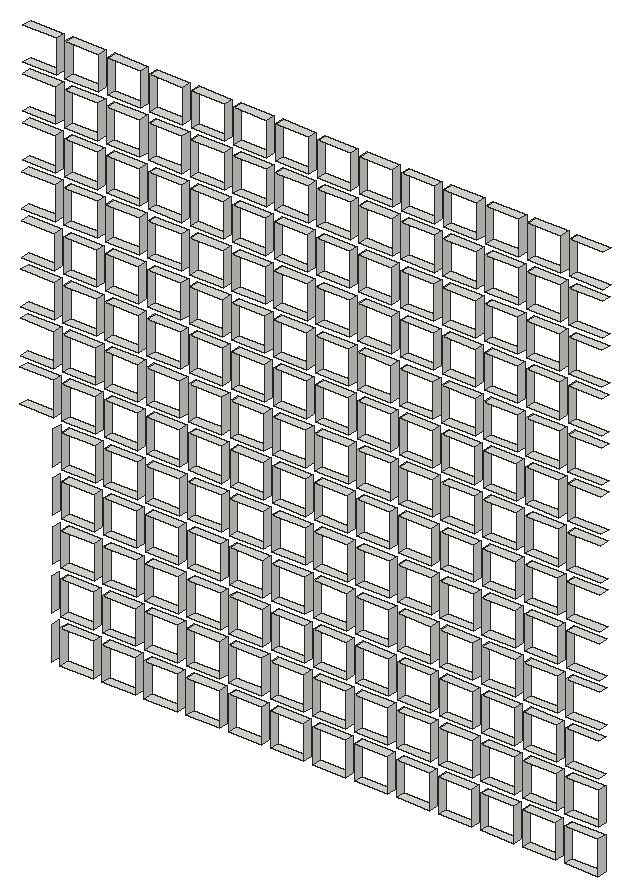
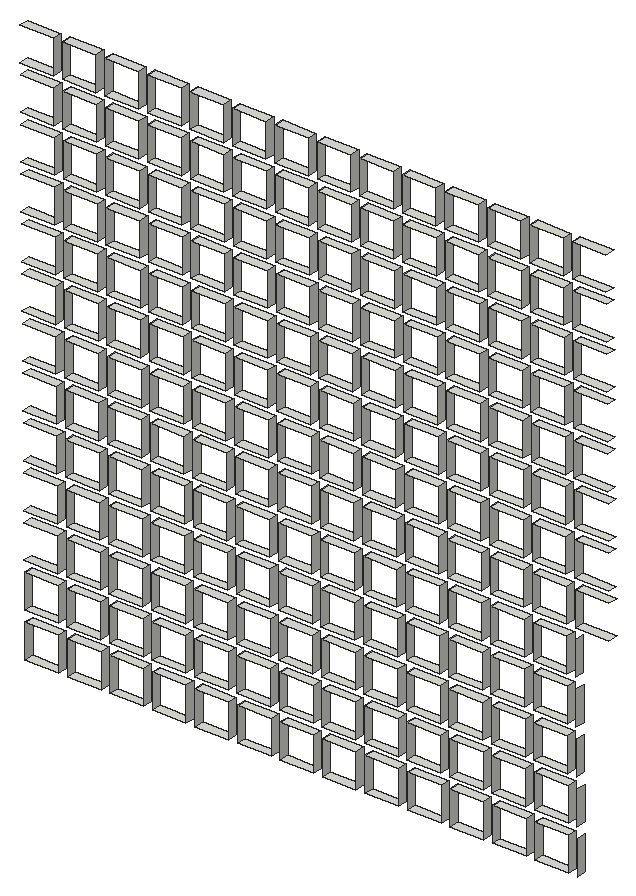
# SketchUp Ruby script. Lengths in inches.
U = 1.inch
M = Sketchup.active_model
def pt(a) = Geom::Point3d.new(a.map { |v| v * U })
def face(e, loops, mat)
  f = e.add_face(loops[0].map { |a| pt(a) })
  loops[1..].each { |l| e.add_face(l.map { |a| pt(a) }).erase! }
  f.material = f.back_material = mat if mat
  f
end
# faces: each face lists its corners as indices into pts; further lists are holes
def faces(e, pts, list, mat = nil) = list.each { |f| face(e, (f[0].is_a?(Array) ? f : [f]).map { |l| l.map { |i| pts[i] } }, mat) }
# xy, xz, yz: faces in a plane at the given z, y or x. An outline is a flat list of corners, or four numbers for a rectangle; further outlines are holes
def ring(l) = l.size == 4 ? [[l[0], l[1]], [l[2], l[1]], [l[2], l[3]], [l[0], l[3]]] : l.each_slice(2).to_a
def flat(e, list, mat, &to3) = list.each { |f| face(e, (f[0].is_a?(Array) ? f : [f]).map { |l| ring(l).map { |u, v| to3.(u, v) } }, mat) }
def xy(e, z, list, mat = nil) = flat(e, list, mat) { |x, y| [x, y, z] }
def xz(e, y, list, mat = nil) = flat(e, list, mat) { |x, z| [x, y, z] }
def yz(e, x, list, mat = nil) = flat(e, list, mat) { |y, z| [x, y, z] }
def lines(e, pts, list) = list.each { |a, b| e.add_line(pt(pts[a]), pt(pts[b])) }
# prism: a flat outline (further loops are holes) pulled along v
def prism(e, loops, v, mat = nil)
  f = face(e, loops, mat); d = Geom::Vector3d.new(v.map { |x| x * U })
  f.pushpull(f.normal.samedirection?(d) ? d.length : -d.length)
end
def box(e, o, s, mat = nil) = prism(e, [[o, [o[0] + s[0], o[1], o[2]], [o[0] + s[0], o[1] + s[1], o[2]], [o[0], o[1] + s[1], o[2]]]], [0, 0, s[2]], mat)
def at(x, y, z, deg = 0) = Geom::Transformation.translation(pt([x, y, z])) * Geom::Transformation.rotation(ORIGIN, Z_AXIS, deg.degrees)
def axes(o, x, y, z) = Geom::Transformation.new([*x, 0, *y, 0, *z, 0, *pt(o).to_a, 1])
def part(name) = M.definitions.add(name)
# library, detail: a bought-in or finely detailed component or shape, given as its bounding box
def library(name, o, s) = part(name).tap { |d| box(d.entities, o, s) }
def detail(e, o, s) = box(e.add_group.entities, o, s)
def put(e, d, t, mat = nil) = e.add_instance(d, t).tap { |i| i.material = mat if mat }
def group(e, t, mat = nil) = e.add_group.tap { |g| g.transformation = t; g.material = mat if mat }.entities
root = M.entities
xy(root,265.77,[[2217.37,480.14,2219.68,480.77],[2220.28,480.14,2222.59,480.77],[2223.19,480.14,2225.5,480.77],[2226.1,480.14,2228.42,480.77],[2229.02,480.14,2231.33,480.77],
  [2231.93,480.14,2234.24,480.77],[2234.84,480.14,2237.15,480.77],[2237.75,480.14,2240.06,480.77],[2240.66,480.14,2242.98,480.77],[2243.58,480.14,2245.89,480.77],
  [2246.49,480.14,2248.8,480.77],[2249.4,480.14,2251.71,480.77],[2252.3125,480.14,2254.625,480.77]])
xy(root,268.09,[[2217.37,480.14,2219.68,480.77],[2220.28,480.14,2222.59,480.77],[2223.19,480.14,2225.5,480.77],[2226.1,480.14,2228.42,480.77],[2229.02,480.14,2231.33,480.77],
  [2231.93,480.14,2234.24,480.77],[2234.84,480.14,2237.15,480.77],[2237.75,480.14,2240.06,480.77],[2240.66,480.14,2242.98,480.77],[2243.58,480.14,2245.89,480.77],
  [2246.49,480.14,2248.8,480.77],[2249.4,480.14,2251.71,480.77],[2252.3125,480.14,2254.625,480.77]])
xy(root,268.82,[[2217.4,480.14,2219.71,480.77],[2220.31,480.14,2222.62,480.77],[2223.22,480.14,2225.53,480.77],[2226.13,480.14,2228.45,480.77],[2229.05,480.14,2231.36,480.77],
  [2231.96,480.14,2234.27,480.77],[2234.87,480.14,2237.18,480.77],[2237.78,480.14,2240.09,480.77],[2240.69,480.14,2243.01,480.77],[2243.61,480.14,2245.92,480.77],
  [2246.52,480.14,2248.83,480.77],[2249.43,480.14,2251.74,480.77],[2252.34,480.14,2254.65,480.77]])
xy(root,271.13,[[2217.4,480.14,2219.71,480.77],[2220.31,480.14,2222.62,480.77],[2223.22,480.14,2225.53,480.77],[2226.13,480.14,2228.45,480.77],[2229.05,480.14,2231.36,480.77],
  [2231.96,480.14,2234.27,480.77],[2234.87,480.14,2237.18,480.77],[2237.78,480.14,2240.09,480.77],[2240.69,480.14,2243.01,480.77],[2243.61,480.14,2245.92,480.77],
  [2246.52,480.14,2248.83,480.77],[2249.43,480.14,2251.74,480.77],[2252.34,480.14,2254.65,480.77]])
xy(root,271.86,[[2217.43,480.14,2219.74,480.77],[2220.34,480.14,2222.65,480.77],[2223.25,480.14,2225.5625,480.77],[2226.16,480.14,2228.47,480.77],[2229.07,480.14,2231.39,480.77],
  [2231.99,480.14,2234.3,480.77],[2234.9,480.14,2237.21,480.77],[2237.81,480.14,2240.12,480.77],[2240.72,480.14,2243.03,480.77],[2243.63,480.14,2245.95,480.77],
  [2246.55,480.14,2248.86,480.77],[2249.46,480.14,2251.77,480.77],[2252.37,480.14,2254.68,480.77]])
xy(root,274.17,[[2217.43,480.14,2219.74,480.77],[2220.34,480.14,2222.65,480.77],[2223.25,480.14,2225.5625,480.77],[2226.16,480.14,2228.47,480.77],[2229.07,480.14,2231.39,480.77],
  [2231.99,480.14,2234.3,480.77],[2234.9,480.14,2237.21,480.77],[2237.81,480.14,2240.12,480.77],[2240.72,480.14,2243.03,480.77],[2243.63,480.14,2245.95,480.77],
  [2246.55,480.14,2248.86,480.77],[2249.46,480.14,2251.77,480.77],[2252.37,480.14,2254.68,480.77]])
xy(root,274.91,[[2217.46,480.14,2219.77,480.77],[2220.37,480.14,2222.68,480.77],[2223.28,480.14,2225.59,480.77],[2226.19,480.14,2228.5,480.77],[2229.1,480.14,2231.42,480.77],
  [2232.02,480.14,2234.33,480.77],[2234.93,480.14,2237.24,480.77],[2237.84,480.14,2240.15,480.77],[2240.75,480.14,2243.0625,480.77],[2243.66,480.14,2245.98,480.77],
  [2246.58,480.14,2248.89,480.77],[2249.49,480.14,2251.8,480.77],[2252.4,480.14,2254.71,480.77]])
xy(root,277.22,[[2217.46,480.14,2219.77,480.77],[2220.37,480.14,2222.68,480.77],[2223.28,480.14,2225.59,480.77],[2226.19,480.14,2228.5,480.77],[2229.1,480.14,2231.42,480.77],
  [2232.02,480.14,2234.33,480.77],[2234.93,480.14,2237.24,480.77],[2237.84,480.14,2240.15,480.77],[2240.75,480.14,2243.0625,480.77],[2243.66,480.14,2245.98,480.77],
  [2246.58,480.14,2248.89,480.77],[2249.49,480.14,2251.8,480.77],[2252.4,480.14,2254.71,480.77]])
xy(root,277.95,[[2217.48,480.14,2219.8,480.77],[2220.4,480.14,2222.71,480.77],[2223.31,480.14,2225.62,480.77],[2226.22,480.14,2228.53,480.77],[2229.13,480.14,2231.44,480.77],
  [2232.04,480.14,2234.36,480.77],[2234.96,480.14,2237.27,480.77],[2237.87,480.14,2240.18,480.77],[2240.78,480.14,2243.09,480.77],[2243.69,480.14,2246,480.77],
  [2246.6,480.14,2248.92,480.77],[2249.52,480.14,2251.83,480.77],[2252.43,480.14,2254.74,480.77]])
xy(root,280.26,[[2217.48,480.14,2219.8,480.77],[2220.4,480.14,2222.71,480.77],[2223.31,480.14,2225.62,480.77],[2226.22,480.14,2228.53,480.77],[2229.13,480.14,2231.44,480.77],
  [2232.04,480.14,2234.36,480.77],[2234.96,480.14,2237.27,480.77],[2237.87,480.14,2240.18,480.77],[2240.78,480.14,2243.09,480.77],[2243.69,480.14,2246,480.77],
  [2246.6,480.14,2248.92,480.77],[2249.52,480.14,2251.83,480.77],[2252.43,480.14,2254.74,480.77]])
xy(root,281,[[2214.6,480.14,2216.91,480.77],[2217.51,480.14,2219.83,480.77],[2220.43,480.14,2222.74,480.77],[2223.34,480.14,2225.65,480.77],[2226.25,480.14,2228.5625,480.77],
  [2229.16,480.14,2231.47,480.77],[2232.07,480.14,2234.39,480.77],[2234.99,480.14,2237.3,480.77],[2237.9,480.14,2240.21,480.77],[2240.81,480.14,2243.12,480.77],
  [2243.72,480.14,2246.03,480.77],[2246.63,480.14,2248.95,480.77],[2249.55,480.14,2251.86,480.77],[2252.46,480.14,2254.77,480.77]])
xy(root,283.31,[[2214.6,480.14,2216.91,480.77],[2217.51,480.14,2219.83,480.77],[2220.43,480.14,2222.74,480.77],[2223.34,480.14,2225.65,480.77],[2226.25,480.14,2228.5625,480.77],
  [2229.16,480.14,2231.47,480.77],[2232.07,480.14,2234.39,480.77],[2234.99,480.14,2237.3,480.77],[2237.9,480.14,2240.21,480.77],[2240.81,480.14,2243.12,480.77],
  [2243.72,480.14,2246.03,480.77],[2246.63,480.14,2248.95,480.77],[2249.55,480.14,2251.86,480.77],[2252.46,480.14,2254.77,480.77]])
xy(root,284.04,[[2214.63,480.14,2216.94,480.77],[2217.54,480.14,2219.85,480.77],[2220.45,480.14,2222.77,480.77],[2223.37,480.14,2225.68,480.77],[2226.28,480.14,2228.59,480.77],
  [2229.19,480.14,2231.5,480.77],[2232.1,480.14,2234.41,480.77],[2235.01,480.14,2237.33,480.77],[2237.93,480.14,2240.24,480.77],[2240.84,480.14,2243.15,480.77],
  [2243.75,480.14,2246.0625,480.77],[2246.66,480.14,2248.97,480.77],[2249.57,480.14,2251.89,480.77],[2252.49,480.14,2254.8,480.77]])
xy(root,286.35,[[2214.63,480.14,2216.94,480.77],[2217.54,480.14,2219.85,480.77],[2220.45,480.14,2222.77,480.77],[2223.37,480.14,2225.68,480.77],[2226.28,480.14,2228.59,480.77],
  [2229.19,480.14,2231.5,480.77],[2232.1,480.14,2234.41,480.77],[2235.01,480.14,2237.33,480.77],[2237.93,480.14,2240.24,480.77],[2240.84,480.14,2243.15,480.77],
  [2243.75,480.14,2246.0625,480.77],[2246.66,480.14,2248.97,480.77],[2249.57,480.14,2251.89,480.77],[2252.49,480.14,2254.8,480.77]])
xy(root,287.09,[[2214.66,480.14,2216.97,480.77],[2217.57,480.14,2219.88,480.77],[2220.48,480.14,2222.8,480.77],[2223.4,480.14,2225.71,480.77],[2226.31,480.14,2228.62,480.77],
  [2229.22,480.14,2231.53,480.77],[2232.13,480.14,2234.44,480.77],[2235.04,480.14,2237.36,480.77],[2237.96,480.14,2240.27,480.77],[2240.87,480.14,2243.18,480.77],
  [2243.78,480.14,2246.09,480.77],[2246.69,480.14,2249,480.77],[2249.6,480.14,2251.92,480.77],[2252.52,480.14,2254.83,480.77]])
xy(root,289.4,[[2214.66,480.14,2216.97,480.77],[2217.57,480.14,2219.88,480.77],[2220.48,480.14,2222.8,480.77],[2223.4,480.14,2225.71,480.77],[2226.31,480.14,2228.62,480.77],
  [2229.22,480.14,2231.53,480.77],[2232.13,480.14,2234.44,480.77],[2235.04,480.14,2237.36,480.77],[2237.96,480.14,2240.27,480.77],[2240.87,480.14,2243.18,480.77],
  [2243.78,480.14,2246.09,480.77],[2246.69,480.14,2249,480.77],[2249.6,480.14,2251.92,480.77],[2252.52,480.14,2254.83,480.77]])
xy(root,290.13,[[2214.6875,480.14,2217,480.77],[2217.6,480.14,2219.91,480.77],[2220.51,480.14,2222.82,480.77],[2223.42,480.14,2225.74,480.77],[2226.34,480.14,2228.65,480.77],
  [2229.25,480.14,2231.5625,480.77],[2232.16,480.14,2234.47,480.77],[2235.07,480.14,2237.38,480.77],[2237.98,480.14,2240.3,480.77],[2240.9,480.14,2243.21,480.77],
  [2243.81,480.14,2246.12,480.77],[2246.72,480.14,2249.03,480.77],[2249.63,480.14,2251.94,480.77],[2252.54,480.14,2254.86,480.77]])
xy(root,292.44,[[2214.6875,480.14,2217,480.77],[2217.6,480.14,2219.91,480.77],[2220.51,480.14,2222.82,480.77],[2223.42,480.14,2225.74,480.77],[2226.34,480.14,2228.65,480.77],
  [2229.25,480.14,2231.5625,480.77],[2232.16,480.14,2234.47,480.77],[2235.07,480.14,2237.38,480.77],[2237.98,480.14,2240.3,480.77],[2240.9,480.14,2243.21,480.77],
  [2243.81,480.14,2246.12,480.77],[2246.72,480.14,2249.03,480.77],[2249.63,480.14,2251.94,480.77],[2252.54,480.14,2254.86,480.77]])
xy(root,293.18,[[2214.72,480.14,2217.03,480.77],[2217.63,480.14,2219.94,480.77],[2220.54,480.14,2222.85,480.77],[2223.45,480.14,2225.77,480.77],[2226.37,480.14,2228.68,480.77],
  [2229.28,480.14,2231.59,480.77],[2232.1875,480.14,2234.5,480.77],[2235.1,480.14,2237.41,480.77],[2238.01,480.14,2240.33,480.77],[2240.93,480.14,2243.24,480.77],
  [2243.84,480.14,2246.15,480.77],[2246.75,480.14,2249.0625,480.77],[2249.66,480.14,2251.97,480.77],[2252.57,480.14,2254.89,480.77]])
xy(root,295.49,[[2214.72,480.14,2217.03,480.77],[2217.63,480.14,2219.94,480.77],[2220.54,480.14,2222.85,480.77],[2223.45,480.14,2225.77,480.77],[2226.37,480.14,2228.68,480.77],
  [2229.28,480.14,2231.59,480.77],[2232.1875,480.14,2234.5,480.77],[2235.1,480.14,2237.41,480.77],[2238.01,480.14,2240.33,480.77],[2240.93,480.14,2243.24,480.77],
  [2243.84,480.14,2246.15,480.77],[2246.75,480.14,2249.0625,480.77],[2249.66,480.14,2251.97,480.77],[2252.57,480.14,2254.89,480.77]])
xy(root,296.22,[[2214.75,480.14,2217.06,480.77],[2217.66,480.14,2219.97,480.77],[2220.57,480.14,2222.88,480.77],[2223.48,480.14,2225.79,480.77],[2226.39,480.14,2228.71,480.77],
  [2229.31,480.14,2231.62,480.77],[2232.22,480.14,2234.53,480.77],[2235.13,480.14,2237.44,480.77],[2238.04,480.14,2240.35,480.77],[2240.95,480.14,2243.27,480.77],
  [2243.87,480.14,2246.18,480.77],[2246.78,480.14,2249.09,480.77],[2249.69,480.14,2252,480.77],[2252.6,480.14,2254.91,480.77]])
xy(root,298.53,[[2214.75,480.14,2217.06,480.77],[2217.66,480.14,2219.97,480.77],[2220.57,480.14,2222.88,480.77],[2223.48,480.14,2225.79,480.77],[2226.39,480.14,2228.71,480.77],
  [2229.31,480.14,2231.62,480.77],[2232.22,480.14,2234.53,480.77],[2235.13,480.14,2237.44,480.77],[2238.04,480.14,2240.35,480.77],[2240.95,480.14,2243.27,480.77],
  [2243.87,480.14,2246.18,480.77],[2246.78,480.14,2249.09,480.77],[2249.69,480.14,2252,480.77],[2252.6,480.14,2254.91,480.77]])
xy(root,299.27,[[2214.78,480.14,2217.09,480.77],[2217.6875,480.14,2220,480.77],[2220.6,480.14,2222.91,480.77],[2223.51,480.14,2225.82,480.77],[2226.42,480.14,2228.74,480.77],
  [2229.34,480.14,2231.65,480.77],[2232.25,480.14,2234.56,480.77],[2235.16,480.14,2237.47,480.77],[2238.07,480.14,2240.38,480.77],[2240.98,480.14,2243.3,480.77],
  [2243.9,480.14,2246.21,480.77],[2246.81,480.14,2249.12,480.77],[2249.72,480.14,2252.03,480.77],[2252.63,480.14,2254.94,480.77]])
xy(root,301.58,[[2214.78,480.14,2217.09,480.77],[2217.6875,480.14,2220,480.77],[2220.6,480.14,2222.91,480.77],[2223.51,480.14,2225.82,480.77],[2226.42,480.14,2228.74,480.77],
  [2229.34,480.14,2231.65,480.77],[2232.25,480.14,2234.56,480.77],[2235.16,480.14,2237.47,480.77],[2238.07,480.14,2240.38,480.77],[2240.98,480.14,2243.3,480.77],
  [2243.9,480.14,2246.21,480.77],[2246.81,480.14,2249.12,480.77],[2249.72,480.14,2252.03,480.77],[2252.63,480.14,2254.94,480.77]])
xy(root,302.31,[[2214.8,480.14,2217.12,480.77],[2217.72,480.14,2220.03,480.77],[2220.63,480.14,2222.94,480.77],[2223.54,480.14,2225.85,480.77],[2226.45,480.14,2228.76,480.77],
  [2229.36,480.14,2231.68,480.77],[2232.28,480.14,2234.59,480.77],[2235.1875,480.14,2237.5,480.77],[2238.1,480.14,2240.41,480.77],[2241.01,480.14,2243.32,480.77],
  [2243.92,480.14,2246.24,480.77],[2246.84,480.14,2249.15,480.77],[2249.75,480.14,2252.0625,480.77],[2252.66,480.14,2254.97,480.77]])
xy(root,304.62,[[2214.8,480.14,2217.12,480.77],[2217.72,480.14,2220.03,480.77],[2220.63,480.14,2222.94,480.77],[2223.54,480.14,2225.85,480.77],[2226.45,480.14,2228.76,480.77],
  [2229.36,480.14,2231.68,480.77],[2232.28,480.14,2234.59,480.77],[2235.1875,480.14,2237.5,480.77],[2238.1,480.14,2240.41,480.77],[2241.01,480.14,2243.32,480.77],
  [2243.92,480.14,2246.24,480.77],[2246.84,480.14,2249.15,480.77],[2249.75,480.14,2252.0625,480.77],[2252.66,480.14,2254.97,480.77]])
yz(root,2216.77,[[480.14,265.77,480.77,268.09]])
yz(root,2216.8,[[480.14,268.82,480.77,271.13]])
yz(root,2216.83,[[480.14,271.86,480.77,274.17]])
yz(root,2216.86,[[480.14,274.91,480.77,277.22]])
yz(root,2216.88,[[480.14,277.95,480.77,280.26]])
yz(root,2216.91,[[480.14,281,480.77,283.31]])
yz(root,2216.94,[[480.14,284.04,480.77,286.35]])
yz(root,2216.97,[[480.14,287.09,480.77,289.4]])
yz(root,2217,[[480.14,290.13,480.77,292.44]])
yz(root,2217.03,[[480.14,293.18,480.77,295.49]])
yz(root,2217.06,[[480.14,296.22,480.77,298.53]])
yz(root,2217.09,[[480.14,299.27,480.77,301.58]])
yz(root,2217.12,[[480.14,302.31,480.77,304.62]])
yz(root,2217.37,[[480.14,265.77,480.77,268.09]])
yz(root,2217.4,[[480.14,268.82,480.77,271.13]])
yz(root,2217.43,[[480.14,271.86,480.77,274.17]])
yz(root,2217.46,[[480.14,274.91,480.77,277.22]])
yz(root,2217.48,[[480.14,277.95,480.77,280.26]])
yz(root,2217.51,[[480.14,281,480.77,283.31]])
yz(root,2217.54,[[480.14,284.04,480.77,286.35]])
yz(root,2217.57,[[480.14,287.09,480.77,289.4]])
yz(root,2217.6,[[480.14,290.13,480.77,292.44]])
yz(root,2217.63,[[480.14,293.18,480.77,295.49]])
yz(root,2217.66,[[480.14,296.22,480.77,298.53]])
yz(root,2217.6875,[[480.14,299.27,480.77,301.58]])
yz(root,2217.72,[[480.14,302.31,480.77,304.62]])
yz(root,2219.68,[[480.14,265.77,480.77,268.09]])
yz(root,2219.71,[[480.14,268.82,480.77,271.13]])
yz(root,2219.74,[[480.14,271.86,480.77,274.17]])
yz(root,2219.77,[[480.14,274.91,480.77,277.22]])
yz(root,2219.8,[[480.14,277.95,480.77,280.26]])
yz(root,2219.83,[[480.14,281,480.77,283.31]])
yz(root,2219.85,[[480.14,284.04,480.77,286.35]])
yz(root,2219.88,[[480.14,287.09,480.77,289.4]])
yz(root,2219.91,[[480.14,290.13,480.77,292.44]])
yz(root,2219.94,[[480.14,293.18,480.77,295.49]])
yz(root,2219.97,[[480.14,296.22,480.77,298.53]])
yz(root,2220,[[480.14,299.27,480.77,301.58]])
yz(root,2220.03,[[480.14,302.31,480.77,304.62]])
yz(root,2220.28,[[480.14,265.77,480.77,268.09]])
yz(root,2220.31,[[480.14,268.82,480.77,271.13]])
yz(root,2220.34,[[480.14,271.86,480.77,274.17]])
yz(root,2220.37,[[480.14,274.91,480.77,277.22]])
yz(root,2220.4,[[480.14,277.95,480.77,280.26]])
yz(root,2220.43,[[480.14,281,480.77,283.31]])
yz(root,2220.45,[[480.14,284.04,480.77,286.35]])
yz(root,2220.48,[[480.14,287.09,480.77,289.4]])
yz(root,2220.51,[[480.14,290.13,480.77,292.44]])
yz(root,2220.54,[[480.14,293.18,480.77,295.49]])
yz(root,2220.57,[[480.14,296.22,480.77,298.53]])
yz(root,2220.6,[[480.14,299.27,480.77,301.58]])
yz(root,2220.63,[[480.14,302.31,480.77,304.62]])
yz(root,2222.59,[[480.14,265.77,480.77,268.09]])
yz(root,2222.62,[[480.14,268.82,480.77,271.13]])
yz(root,2222.65,[[480.14,271.86,480.77,274.17]])
yz(root,2222.68,[[480.14,274.91,480.77,277.22]])
yz(root,2222.71,[[480.14,277.95,480.77,280.26]])
yz(root,2222.74,[[480.14,281,480.77,283.31]])
yz(root,2222.77,[[480.14,284.04,480.77,286.35]])
yz(root,2222.8,[[480.14,287.09,480.77,289.4]])
yz(root,2222.82,[[480.14,290.13,480.77,292.44]])
yz(root,2222.85,[[480.14,293.18,480.77,295.49]])
yz(root,2222.88,[[480.14,296.22,480.77,298.53]])
yz(root,2222.91,[[480.14,299.27,480.77,301.58]])
yz(root,2222.94,[[480.14,302.31,480.77,304.62]])
yz(root,2223.19,[[480.14,265.77,480.77,268.09]])
yz(root,2223.22,[[480.14,268.82,480.77,271.13]])
yz(root,2223.25,[[480.14,271.86,480.77,274.17]])
yz(root,2223.28,[[480.14,274.91,480.77,277.22]])
yz(root,2223.31,[[480.14,277.95,480.77,280.26]])
yz(root,2223.34,[[480.14,281,480.77,283.31]])
yz(root,2223.37,[[480.14,284.04,480.77,286.35]])
yz(root,2223.4,[[480.14,287.09,480.77,289.4]])
yz(root,2223.42,[[480.14,290.13,480.77,292.44]])
yz(root,2223.45,[[480.14,293.18,480.77,295.49]])
yz(root,2223.48,[[480.14,296.22,480.77,298.53]])
yz(root,2223.51,[[480.14,299.27,480.77,301.58]])
yz(root,2223.54,[[480.14,302.31,480.77,304.62]])
yz(root,2225.5,[[480.14,265.77,480.77,268.09]])
yz(root,2225.53,[[480.14,268.82,480.77,271.13]])
yz(root,2225.5625,[[480.14,271.86,480.77,274.17]])
yz(root,2225.59,[[480.14,274.91,480.77,277.22]])
yz(root,2225.62,[[480.14,277.95,480.77,280.26]])
yz(root,2225.65,[[480.14,281,480.77,283.31]])
yz(root,2225.68,[[480.14,284.04,480.77,286.35]])
yz(root,2225.71,[[480.14,287.09,480.77,289.4]])
yz(root,2225.74,[[480.14,290.13,480.77,292.44]])
yz(root,2225.77,[[480.14,293.18,480.77,295.49]])
yz(root,2225.79,[[480.14,296.22,480.77,298.53]])
yz(root,2225.82,[[480.14,299.27,480.77,301.58]])
yz(root,2225.85,[[480.14,302.31,480.77,304.62]])
yz(root,2226.1,[[480.14,265.77,480.77,268.09]])
yz(root,2226.13,[[480.14,268.82,480.77,271.13]])
yz(root,2226.16,[[480.14,271.86,480.77,274.17]])
yz(root,2226.19,[[480.14,274.91,480.77,277.22]])
yz(root,2226.22,[[480.14,277.95,480.77,280.26]])
yz(root,2226.25,[[480.14,281,480.77,283.31]])
yz(root,2226.28,[[480.14,284.04,480.77,286.35]])
yz(root,2226.31,[[480.14,287.09,480.77,289.4]])
yz(root,2226.34,[[480.14,290.13,480.77,292.44]])
yz(root,2226.37,[[480.14,293.18,480.77,295.49]])
yz(root,2226.39,[[480.14,296.22,480.77,298.53]])
yz(root,2226.42,[[480.14,299.27,480.77,301.58]])
yz(root,2226.45,[[480.14,302.31,480.77,304.62]])
yz(root,2228.42,[[480.14,265.77,480.77,268.09]])
yz(root,2228.45,[[480.14,268.82,480.77,271.13]])
yz(root,2228.47,[[480.14,271.86,480.77,274.17]])
yz(root,2228.5,[[480.14,274.91,480.77,277.22]])
yz(root,2228.53,[[480.14,277.95,480.77,280.26]])
yz(root,2228.5625,[[480.14,281,480.77,283.31]])
yz(root,2228.59,[[480.14,284.04,480.77,286.35]])
yz(root,2228.62,[[480.14,287.09,480.77,289.4]])
yz(root,2228.65,[[480.14,290.13,480.77,292.44]])
yz(root,2228.68,[[480.14,293.18,480.77,295.49]])
yz(root,2228.71,[[480.14,296.22,480.77,298.53]])
yz(root,2228.74,[[480.14,299.27,480.77,301.58]])
yz(root,2228.76,[[480.14,302.31,480.77,304.62]])
yz(root,2229.02,[[480.14,265.77,480.77,268.09]])
yz(root,2229.05,[[480.14,268.82,480.77,271.13]])
yz(root,2229.07,[[480.14,271.86,480.77,274.17]])
yz(root,2229.1,[[480.14,274.91,480.77,277.22]])
yz(root,2229.13,[[480.14,277.95,480.77,280.26]])
yz(root,2229.16,[[480.14,281,480.77,283.31]])
yz(root,2229.19,[[480.14,284.04,480.77,286.35]])
yz(root,2229.22,[[480.14,287.09,480.77,289.4]])
yz(root,2229.25,[[480.14,290.13,480.77,292.44]])
yz(root,2229.28,[[480.14,293.18,480.77,295.49]])
yz(root,2229.31,[[480.14,296.22,480.77,298.53]])
yz(root,2229.34,[[480.14,299.27,480.77,301.58]])
yz(root,2229.36,[[480.14,302.31,480.77,304.62]])
yz(root,2231.33,[[480.14,265.77,480.77,268.09]])
yz(root,2231.36,[[480.14,268.82,480.77,271.13]])
yz(root,2231.39,[[480.14,271.86,480.77,274.17]])
yz(root,2231.42,[[480.14,274.91,480.77,277.22]])
yz(root,2231.44,[[480.14,277.95,480.77,280.26]])
yz(root,2231.47,[[480.14,281,480.77,283.31]])
yz(root,2231.5,[[480.14,284.04,480.77,286.35]])
yz(root,2231.53,[[480.14,287.09,480.77,289.4]])
yz(root,2231.5625,[[480.14,290.13,480.77,292.44]])
yz(root,2231.59,[[480.14,293.18,480.77,295.49]])
yz(root,2231.62,[[480.14,296.22,480.77,298.53]])
yz(root,2231.65,[[480.14,299.27,480.77,301.58]])
yz(root,2231.68,[[480.14,302.31,480.77,304.62]])
yz(root,2231.93,[[480.14,265.77,480.77,268.09]])
yz(root,2231.96,[[480.14,268.82,480.77,271.13]])
yz(root,2231.99,[[480.14,271.86,480.77,274.17]])
yz(root,2232.02,[[480.14,274.91,480.77,277.22]])
yz(root,2232.04,[[480.14,277.95,480.77,280.26]])
yz(root,2232.07,[[480.14,281,480.77,283.31]])
yz(root,2232.1,[[480.14,284.04,480.77,286.35]])
yz(root,2232.13,[[480.14,287.09,480.77,289.4]])
yz(root,2232.16,[[480.14,290.13,480.77,292.44]])
yz(root,2232.1875,[[480.14,293.18,480.77,295.49]])
yz(root,2232.22,[[480.14,296.22,480.77,298.53]])
yz(root,2232.25,[[480.14,299.27,480.77,301.58]])
yz(root,2232.28,[[480.14,302.31,480.77,304.62]])
yz(root,2234.24,[[480.14,265.77,480.77,268.09]])
yz(root,2234.27,[[480.14,268.82,480.77,271.13]])
yz(root,2234.3,[[480.14,271.86,480.77,274.17]])
yz(root,2234.33,[[480.14,274.91,480.77,277.22]])
yz(root,2234.36,[[480.14,277.95,480.77,280.26]])
yz(root,2234.39,[[480.14,281,480.77,283.31]])
yz(root,2234.41,[[480.14,284.04,480.77,286.35]])
yz(root,2234.44,[[480.14,287.09,480.77,289.4]])
yz(root,2234.47,[[480.14,290.13,480.77,292.44]])
yz(root,2234.5,[[480.14,293.18,480.77,295.49]])
yz(root,2234.53,[[480.14,296.22,480.77,298.53]])
yz(root,2234.56,[[480.14,299.27,480.77,301.58]])
yz(root,2234.59,[[480.14,302.31,480.77,304.62]])
yz(root,2234.84,[[480.14,265.77,480.77,268.09]])
yz(root,2234.87,[[480.14,268.82,480.77,271.13]])
yz(root,2234.9,[[480.14,271.86,480.77,274.17]])
yz(root,2234.93,[[480.14,274.91,480.77,277.22]])
yz(root,2234.96,[[480.14,277.95,480.77,280.26]])
yz(root,2234.99,[[480.14,281,480.77,283.31]])
yz(root,2235.01,[[480.14,284.04,480.77,286.35]])
yz(root,2235.04,[[480.14,287.09,480.77,289.4]])
yz(root,2235.07,[[480.14,290.13,480.77,292.44]])
yz(root,2235.1,[[480.14,293.18,480.77,295.49]])
yz(root,2235.13,[[480.14,296.22,480.77,298.53]])
yz(root,2235.16,[[480.14,299.27,480.77,301.58]])
yz(root,2235.1875,[[480.14,302.31,480.77,304.62]])
yz(root,2237.15,[[480.14,265.77,480.77,268.09]])
yz(root,2237.18,[[480.14,268.82,480.77,271.13]])
yz(root,2237.21,[[480.14,271.86,480.77,274.17]])
yz(root,2237.24,[[480.14,274.91,480.77,277.22]])
yz(root,2237.27,[[480.14,277.95,480.77,280.26]])
yz(root,2237.3,[[480.14,281,480.77,283.31]])
yz(root,2237.33,[[480.14,284.04,480.77,286.35]])
yz(root,2237.36,[[480.14,287.09,480.77,289.4]])
yz(root,2237.38,[[480.14,290.13,480.77,292.44]])
yz(root,2237.41,[[480.14,293.18,480.77,295.49]])
yz(root,2237.44,[[480.14,296.22,480.77,298.53]])
yz(root,2237.47,[[480.14,299.27,480.77,301.58]])
yz(root,2237.5,[[480.14,302.31,480.77,304.62]])
yz(root,2237.75,[[480.14,265.77,480.77,268.09]])
yz(root,2237.78,[[480.14,268.82,480.77,271.13]])
yz(root,2237.81,[[480.14,271.86,480.77,274.17]])
yz(root,2237.84,[[480.14,274.91,480.77,277.22]])
yz(root,2237.87,[[480.14,277.95,480.77,280.26]])
yz(root,2237.9,[[480.14,281,480.77,283.31]])
yz(root,2237.93,[[480.14,284.04,480.77,286.35]])
yz(root,2237.96,[[480.14,287.09,480.77,289.4]])
yz(root,2237.98,[[480.14,290.13,480.77,292.44]])
yz(root,2238.01,[[480.14,293.18,480.77,295.49]])
yz(root,2238.04,[[480.14,296.22,480.77,298.53]])
yz(root,2238.07,[[480.14,299.27,480.77,301.58]])
yz(root,2238.1,[[480.14,302.31,480.77,304.62]])
yz(root,2240.06,[[480.14,265.77,480.77,268.09]])
yz(root,2240.09,[[480.14,268.82,480.77,271.13]])
yz(root,2240.12,[[480.14,271.86,480.77,274.17]])
yz(root,2240.15,[[480.14,274.91,480.77,277.22]])
yz(root,2240.18,[[480.14,277.95,480.77,280.26]])
yz(root,2240.21,[[480.14,281,480.77,283.31]])
yz(root,2240.24,[[480.14,284.04,480.77,286.35]])
yz(root,2240.27,[[480.14,287.09,480.77,289.4]])
yz(root,2240.3,[[480.14,290.13,480.77,292.44]])
yz(root,2240.33,[[480.14,293.18,480.77,295.49]])
yz(root,2240.35,[[480.14,296.22,480.77,298.53]])
yz(root,2240.38,[[480.14,299.27,480.77,301.58]])
yz(root,2240.41,[[480.14,302.31,480.77,304.62]])
yz(root,2240.66,[[480.14,265.77,480.77,268.09]])
yz(root,2240.69,[[480.14,268.82,480.77,271.13]])
yz(root,2240.72,[[480.14,271.86,480.77,274.17]])
yz(root,2240.75,[[480.14,274.91,480.77,277.22]])
yz(root,2240.78,[[480.14,277.95,480.77,280.26]])
yz(root,2240.81,[[480.14,281,480.77,283.31]])
yz(root,2240.84,[[480.14,284.04,480.77,286.35]])
yz(root,2240.87,[[480.14,287.09,480.77,289.4]])
yz(root,2240.9,[[480.14,290.13,480.77,292.44]])
yz(root,2240.93,[[480.14,293.18,480.77,295.49]])
yz(root,2240.95,[[480.14,296.22,480.77,298.53]])
yz(root,2240.98,[[480.14,299.27,480.77,301.58]])
yz(root,2241.01,[[480.14,302.31,480.77,304.62]])
yz(root,2242.98,[[480.14,265.77,480.77,268.09]])
yz(root,2243.01,[[480.14,268.82,480.77,271.13]])
yz(root,2243.03,[[480.14,271.86,480.77,274.17]])
yz(root,2243.0625,[[480.14,274.91,480.77,277.22]])
yz(root,2243.09,[[480.14,277.95,480.77,280.26]])
yz(root,2243.12,[[480.14,281,480.77,283.31]])
yz(root,2243.15,[[480.14,284.04,480.77,286.35]])
yz(root,2243.18,[[480.14,287.09,480.77,289.4]])
yz(root,2243.21,[[480.14,290.13,480.77,292.44]])
yz(root,2243.24,[[480.14,293.18,480.77,295.49]])
yz(root,2243.27,[[480.14,296.22,480.77,298.53]])
yz(root,2243.3,[[480.14,299.27,480.77,301.58]])
yz(root,2243.32,[[480.14,302.31,480.77,304.62]])
yz(root,2243.58,[[480.14,265.77,480.77,268.09]])
yz(root,2243.61,[[480.14,268.82,480.77,271.13]])
yz(root,2243.63,[[480.14,271.86,480.77,274.17]])
yz(root,2243.66,[[480.14,274.91,480.77,277.22]])
yz(root,2243.69,[[480.14,277.95,480.77,280.26]])
yz(root,2243.72,[[480.14,281,480.77,283.31]])
yz(root,2243.75,[[480.14,284.04,480.77,286.35]])
yz(root,2243.78,[[480.14,287.09,480.77,289.4]])
yz(root,2243.81,[[480.14,290.13,480.77,292.44]])
yz(root,2243.84,[[480.14,293.18,480.77,295.49]])
yz(root,2243.87,[[480.14,296.22,480.77,298.53]])
yz(root,2243.9,[[480.14,299.27,480.77,301.58]])
yz(root,2243.92,[[480.14,302.31,480.77,304.62]])
yz(root,2245.89,[[480.14,265.77,480.77,268.09]])
yz(root,2245.92,[[480.14,268.82,480.77,271.13]])
yz(root,2245.95,[[480.14,271.86,480.77,274.17]])
yz(root,2245.98,[[480.14,274.91,480.77,277.22]])
yz(root,2246,[[480.14,277.95,480.77,280.26]])
yz(root,2246.03,[[480.14,281,480.77,283.31]])
yz(root,2246.0625,[[480.14,284.04,480.77,286.35]])
yz(root,2246.09,[[480.14,287.09,480.77,289.4]])
yz(root,2246.12,[[480.14,290.13,480.77,292.44]])
yz(root,2246.15,[[480.14,293.18,480.77,295.49]])
yz(root,2246.18,[[480.14,296.22,480.77,298.53]])
yz(root,2246.21,[[480.14,299.27,480.77,301.58]])
yz(root,2246.24,[[480.14,302.31,480.77,304.62]])
yz(root,2246.49,[[480.14,265.77,480.77,268.09]])
yz(root,2246.52,[[480.14,268.82,480.77,271.13]])
yz(root,2246.55,[[480.14,271.86,480.77,274.17]])
yz(root,2246.58,[[480.14,274.91,480.77,277.22]])
yz(root,2246.6,[[480.14,277.95,480.77,280.26]])
yz(root,2246.63,[[480.14,281,480.77,283.31]])
yz(root,2246.66,[[480.14,284.04,480.77,286.35]])
yz(root,2246.69,[[480.14,287.09,480.77,289.4]])
yz(root,2246.72,[[480.14,290.13,480.77,292.44]])
yz(root,2246.75,[[480.14,293.18,480.77,295.49]])
yz(root,2246.78,[[480.14,296.22,480.77,298.53]])
yz(root,2246.81,[[480.14,299.27,480.77,301.58]])
yz(root,2246.84,[[480.14,302.31,480.77,304.62]])
yz(root,2248.8,[[480.14,265.77,480.77,268.09]])
yz(root,2248.83,[[480.14,268.82,480.77,271.13]])
yz(root,2248.86,[[480.14,271.86,480.77,274.17]])
yz(root,2248.89,[[480.14,274.91,480.77,277.22]])
yz(root,2248.92,[[480.14,277.95,480.77,280.26]])
yz(root,2248.95,[[480.14,281,480.77,283.31]])
yz(root,2248.97,[[480.14,284.04,480.77,286.35]])
yz(root,2249,[[480.14,287.09,480.77,289.4]])
yz(root,2249.03,[[480.14,290.13,480.77,292.44]])
yz(root,2249.0625,[[480.14,293.18,480.77,295.49]])
yz(root,2249.09,[[480.14,296.22,480.77,298.53]])
yz(root,2249.12,[[480.14,299.27,480.77,301.58]])
yz(root,2249.15,[[480.14,302.31,480.77,304.62]])
yz(root,2249.4,[[480.14,265.77,480.77,268.09]])
yz(root,2249.43,[[480.14,268.82,480.77,271.13]])
yz(root,2249.46,[[480.14,271.86,480.77,274.17]])
yz(root,2249.49,[[480.14,274.91,480.77,277.22]])
yz(root,2249.52,[[480.14,277.95,480.77,280.26]])
yz(root,2249.55,[[480.14,281,480.77,283.31]])
yz(root,2249.57,[[480.14,284.04,480.77,286.35]])
yz(root,2249.6,[[480.14,287.09,480.77,289.4]])
yz(root,2249.63,[[480.14,290.13,480.77,292.44]])
yz(root,2249.66,[[480.14,293.18,480.77,295.49]])
yz(root,2249.69,[[480.14,296.22,480.77,298.53]])
yz(root,2249.72,[[480.14,299.27,480.77,301.58]])
yz(root,2249.75,[[480.14,302.31,480.77,304.62]])
yz(root,2251.71,[[480.14,265.77,480.77,268.09]])
yz(root,2251.74,[[480.14,268.82,480.77,271.13]])
yz(root,2251.77,[[480.14,271.86,480.77,274.17]])
yz(root,2251.8,[[480.14,274.91,480.77,277.22]])
yz(root,2251.83,[[480.14,277.95,480.77,280.26]])
yz(root,2251.86,[[480.14,281,480.77,283.31]])
yz(root,2251.89,[[480.14,284.04,480.77,286.35]])
yz(root,2251.92,[[480.14,287.09,480.77,289.4]])
yz(root,2251.94,[[480.14,290.13,480.77,292.44]])
yz(root,2251.97,[[480.14,293.18,480.77,295.49]])
yz(root,2252,[[480.14,296.22,480.77,298.53]])
yz(root,2252.03,[[480.14,299.27,480.77,301.58]])
yz(root,2252.0625,[[480.14,302.31,480.77,304.62]])
yz(root,2252.3125,[[480.14,265.77,480.77,268.09]])
yz(root,2252.34,[[480.14,268.82,480.77,271.13]])
yz(root,2252.37,[[480.14,271.86,480.77,274.17]])
yz(root,2252.4,[[480.14,274.91,480.77,277.22]])
yz(root,2252.43,[[480.14,277.95,480.77,280.26]])
yz(root,2252.46,[[480.14,281,480.77,283.31]])
yz(root,2252.49,[[480.14,284.04,480.77,286.35]])
yz(root,2252.52,[[480.14,287.09,480.77,289.4]])
yz(root,2252.54,[[480.14,290.13,480.77,292.44]])
yz(root,2252.57,[[480.14,293.18,480.77,295.49]])
yz(root,2252.6,[[480.14,296.22,480.77,298.53]])
yz(root,2252.63,[[480.14,299.27,480.77,301.58]])
yz(root,2252.66,[[480.14,302.31,480.77,304.62]])
yz(root,2254.625,[[480.14,265.77,480.77,268.09]])
yz(root,2254.65,[[480.14,268.82,480.77,271.13]])
